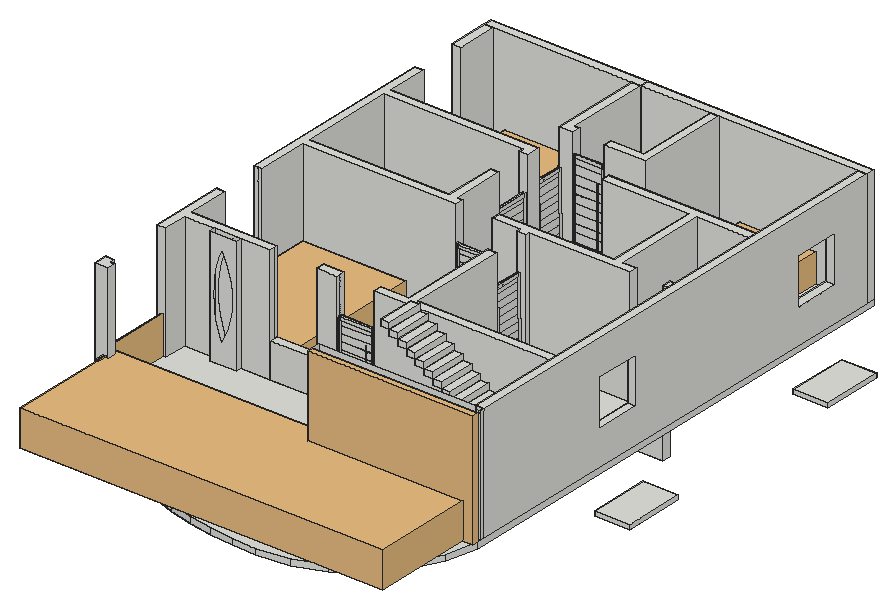
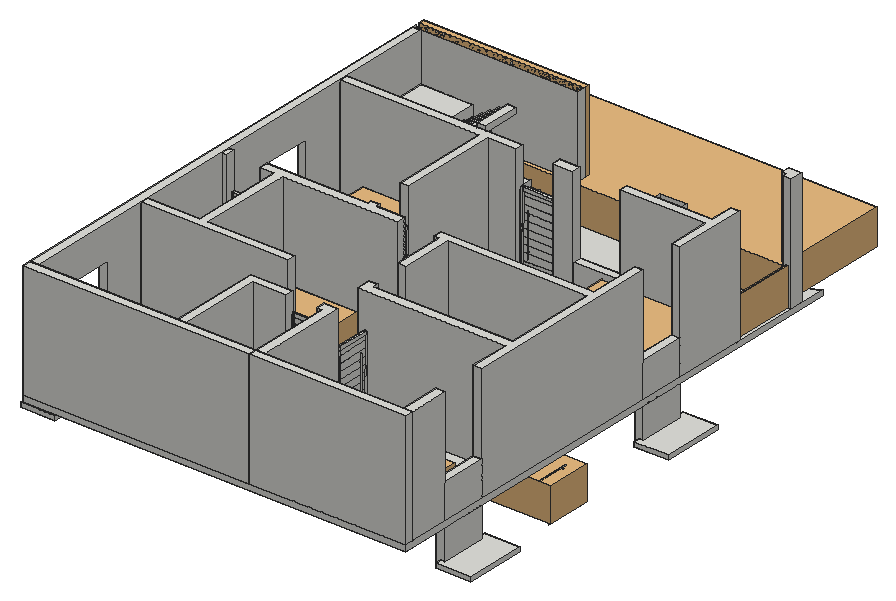
# SketchUp Ruby script. Lengths in inches.
U = 1.inch
M = Sketchup.active_model
def pt(a) = Geom::Point3d.new(a.map { |v| v * U })
def face(e, loops, mat)
  f = e.add_face(loops[0].map { |a| pt(a) })
  loops[1..].each { |l| e.add_face(l.map { |a| pt(a) }).erase! }
  f.material = f.back_material = mat if mat
  f
end
# faces: each face lists its corners as indices into pts; further lists are holes
def faces(e, pts, list, mat = nil) = list.each { |f| face(e, (f[0].is_a?(Array) ? f : [f]).map { |l| l.map { |i| pts[i] } }, mat) }
# xy, xz, yz: faces in a plane at the given z, y or x. An outline is a flat list of corners, or four numbers for a rectangle; further outlines are holes
def ring(l) = l.size == 4 ? [[l[0], l[1]], [l[2], l[1]], [l[2], l[3]], [l[0], l[3]]] : l.each_slice(2).to_a
def flat(e, list, mat, &to3) = list.each { |f| face(e, (f[0].is_a?(Array) ? f : [f]).map { |l| ring(l).map { |u, v| to3.(u, v) } }, mat) }
def xy(e, z, list, mat = nil) = flat(e, list, mat) { |x, y| [x, y, z] }
def xz(e, y, list, mat = nil) = flat(e, list, mat) { |x, z| [x, y, z] }
def yz(e, x, list, mat = nil) = flat(e, list, mat) { |y, z| [x, y, z] }
def lines(e, pts, list) = list.each { |a, b| e.add_line(pt(pts[a]), pt(pts[b])) }
# prism: a flat outline (further loops are holes) pulled along v
def prism(e, loops, v, mat = nil)
  f = face(e, loops, mat); d = Geom::Vector3d.new(v.map { |x| x * U })
  f.pushpull(f.normal.samedirection?(d) ? d.length : -d.length)
end
def box(e, o, s, mat = nil) = prism(e, [[o, [o[0] + s[0], o[1], o[2]], [o[0] + s[0], o[1] + s[1], o[2]], [o[0], o[1] + s[1], o[2]]]], [0, 0, s[2]], mat)
def at(x, y, z, deg = 0) = Geom::Transformation.translation(pt([x, y, z])) * Geom::Transformation.rotation(ORIGIN, Z_AXIS, deg.degrees)
def axes(o, x, y, z) = Geom::Transformation.new([*x, 0, *y, 0, *z, 0, *pt(o).to_a, 1])
def part(name) = M.definitions.add(name)
# library, detail: a bought-in or finely detailed component or shape, given as its bounding box
def library(name, o, s) = part(name).tap { |d| box(d.entities, o, s) }
def detail(e, o, s) = box(e.add_group.entities, o, s)
def put(e, d, t, mat = nil) = e.add_instance(d, t).tap { |i| i.material = mat if mat }
def group(e, t, mat = nil) = e.add_group.tap { |g| g.transformation = t; g.material = mat if mat }.entities
root = M.entities
c1 = part("Группа\#62")
xz(c1.entities,1.5625,[[-122.05,-1.18,-77.55,0]])
p = [[-122.05,0,0],[-122.05,1.5625,0]]
lines(c1.entities,p,[[0,1]])
c2 = part("Группа\#121")
xz(c2.entities,0,[[[0,0,3.9375,3.9375],[0.39,0.39,3.54,3.54]]])
p = [[0.39,0,0.39],[1.97,0.39,1.97],[3.54,0,0.39],[0.39,0,3.54],[3.54,0,3.54]]
faces(c2.entities,p,[[0,1,2],[0,3,1],[4,2,1],[4,1,3]])
c3 = part("Группа\#115")
xy(c3.entities,0,[[0,-1.97,3.9375,9.84]])
xy(c3.entities,7.875,[[0,-1.97,3.9375,13.78]])
xz(c3.entities,-1.97,[[0,0,3.9375,7.875]])
yz(c3.entities,0,[[-1.97,0,-1.97,7.875,13.78,7.875,13.78,3.9375,13.3,3.81,12.84,3.65,12.4,3.4375,11.98,3.18,11.58,2.89,11.22,2.56,10.89,2.19,10.6,1.8,10.34,1.38,10.13,0.9375,9.96,0.48,9.84,0]])
yz(c3.entities,3.9375,[[-1.97,0,9.84,0,9.96,0.48,10.13,0.9375,10.34,1.38,10.6,1.8,10.89,2.19,11.22,2.56,11.58,2.89,11.98,3.18,12.4,3.4375,12.84,3.65,13.3,3.81,13.78,3.9375,13.78,7.875,-1.97,7.875]])
p = [[0,9.84,0],[0,9.96,0.48],[3.9375,9.96,0.48],[3.9375,9.84,0],[0,10.13,0.9375],[3.9375,10.13,0.9375],
  [0,10.34,1.38],[3.9375,10.34,1.38],[0,10.6,1.8],[3.9375,10.6,1.8],[0,10.89,2.19],[3.9375,10.89,2.19],
  [0,11.22,2.56],[3.9375,11.22,2.56],[0,11.58,2.89],[3.9375,11.58,2.89],[0,11.98,3.18],[3.9375,11.98,3.18],
  [0,12.4,3.4375],[3.9375,12.4,3.4375],[0,12.84,3.65],[3.9375,12.84,3.65],[0,13.3,3.81],[3.9375,13.3,3.81],
  [0,13.78,3.9375],[3.9375,13.78,3.9375]]
faces(c3.entities,p,[[0,1,2,3],[1,4,5,2],[4,6,7,5],[6,8,9,7],[8,10,11,9],[10,12,13,11],[12,14,15,13],[14,16,17,15],
  [16,18,19,17],[18,20,21,19],[20,22,23,21],[22,24,25,23]])
put(c3.entities,c2,at(0,13.78,3.9375))
c4 = library("Группа\#83",[-9.65,-17.52,0],[19.3,35.04,0.98])
c5 = library("Группа\#64",[-11.61,-17.52,0],[23.22,35.04,0.98])
c6 = part("Группа\#82")
xy(c6.entities,0,[[[-5.71,-17.52,5.71,17.52],[-3.66,-15.47,3.66,15.47]]])
xy(c6.entities,0.49,[[-3.35,-15.16,3.35,15.16]])
xy(c6.entities,0.98,[[[-5.71,-17.52,5.71,17.52],[-3.66,-15.47,3.66,15.47]]])
xz(c6.entities,-17.52,[[-5.71,0,5.71,0.98]])
xz(c6.entities,-15.16,[[-3.35,0.31,3.35,0.49],[-3.35,0.49,3.35,0.67]])
xz(c6.entities,15.16,[[-3.35,0.31,3.35,0.49],[-3.35,0.49,3.35,0.67]])
xz(c6.entities,17.52,[[-5.71,0,5.71,0.98]])
yz(c6.entities,-5.71,[[-17.52,0,17.52,0.98]])
yz(c6.entities,-3.35,[[-15.16,0.31,15.16,0.49],[-15.16,0.49,15.16,0.67]])
yz(c6.entities,3.35,[[-15.16,0.31,15.16,0.49],[-15.16,0.49,15.16,0.67]])
yz(c6.entities,5.71,[[-17.52,0,17.52,0.98]])
p = [[-3.35,-15.16,0.31],[3.35,-15.16,0.31],[-3.66,-15.47,0],[-3.66,15.47,0],[3.66,-15.47,0],[3.35,15.16,0.31],
  [3.66,15.47,0],[-3.35,15.16,0.31],[-3.35,-15.16,0.67],[-3.35,15.16,0.67],[-3.66,-15.47,0.98],[3.66,-15.47,0.98],
  [-3.66,15.47,0.98],[3.35,-15.16,0.67],[3.35,15.16,0.67],[3.66,15.47,0.98]]
faces(c6.entities,p,[[0,1,2],[2,3,0],[2,1,4],[5,4,1],[6,4,5],[7,0,3],[3,6,7],[5,7,6],
  [8,9,10],[10,11,8],[10,9,12],[13,8,11],[14,13,11],[14,11,15],[15,12,9],[14,15,9]])
c7 = part("Группа\#67")
xy(c7.entities,0,[[[-5.51,-17.52,5.51,17.52],[-3.46,-15.47,3.46,15.47]]])
xy(c7.entities,0.49,[[-3.15,-15.16,3.15,15.16]])
xy(c7.entities,0.98,[[[-5.51,-17.52,5.51,17.52],[-3.46,-15.47,3.46,15.47]]])
xz(c7.entities,-17.52,[[-5.51,0,5.51,0.98]])
xz(c7.entities,-15.16,[[-3.15,0.31,3.15,0.49],[-3.15,0.49,3.15,0.67]])
xz(c7.entities,15.16,[[-3.15,0.31,3.15,0.49],[-3.15,0.49,3.15,0.67]])
xz(c7.entities,17.52,[[-5.51,0,5.51,0.98]])
yz(c7.entities,-5.51,[[-17.52,0,17.52,0.98]])
yz(c7.entities,-3.15,[[-15.16,0.31,15.16,0.49],[-15.16,0.49,15.16,0.67]])
yz(c7.entities,3.15,[[-15.16,0.31,15.16,0.49],[-15.16,0.49,15.16,0.67]])
yz(c7.entities,5.51,[[-17.52,0,17.52,0.98]])
p = [[-3.15,-15.16,0.31],[3.15,-15.16,0.31],[-3.46,-15.47,0],[-3.46,15.47,0],[3.46,-15.47,0],[3.15,15.16,0.31],
  [3.46,15.47,0],[-3.15,15.16,0.31],[-3.15,-15.16,0.67],[-3.15,15.16,0.67],[-3.46,-15.47,0.98],[3.46,-15.47,0.98],
  [-3.46,15.47,0.98],[3.15,-15.16,0.67],[3.15,15.16,0.67],[3.46,15.47,0.98]]
faces(c7.entities,p,[[0,1,2],[2,3,0],[2,1,4],[5,4,1],[6,4,5],[7,0,3],[3,6,7],[5,7,6],
  [8,9,10],[10,11,8],[10,9,12],[13,8,11],[14,13,11],[14,11,15],[15,12,9],[14,15,9]])
c8 = part("Группа\#71")
xy(c8.entities,0,[[-3.05,-15.16,3.05,15.16]])
c9 = part("Group\#141")
box(c9.entities,[0,0,0],[37.68,9,36.625])
c10 = part("Group\#14")
xy(c10.entities,36,[[0,0,9,48]])
yz(c10.entities,0,[[0,0,48,36]])
yz(c10.entities,9,[[0,0,48,36]])
c11 = part("Group\#15")
xy(c11.entities,0,[[0,0,9,48]])
xz(c11.entities,0,[[0,0,9,36]])
xz(c11.entities,48,[[0,0,9,36]])
put(c11.entities,c10,at(0,0,0))
c12 = part("Group\#17")
box(c12.entities,[0,0,0],[36,62.875,4.625])
c13 = library("Group\#5",[0,0,0],[3.15,94.04,36])
c14 = part("Agrupar\#4")
xy(c14.entities,0,[[0,0,60.82,4.875]])
c15 = part("Agrupar\#7")
box(c15.entities,[0,0,0.25],[0.65,5.875,0.35])
c16 = part("Agrupar\#15")
prism(c16.entities,[[[0,0.625,0],[0.65,0.625,0],[0.65,0,0],[0,0,0]]],[0,0.02,45.16])
c17 = part("Agrupar\#14")
put(c17.entities,c15,at(0,0.65,6.88))
put(c17.entities,c16,at(0,0,0))
put(c17.entities,c15,at(0,0.65,40.25))
c18 = part("Agrupar\#6")
prism(c18.entities,[[[-0.5,0.62,-4.9375],[0.77,0.62,-4.9375],[0.77,-0.19,-4.9375],[-0.5,-0.19,-4.9375]]],[0,0.03,52.91])
c19 = part("Agrupar\#8")
put(c19.entities,c15,at(0,0.65,6.88))
put(c19.entities,c18,at(0,0,0))
put(c19.entities,c15,at(0,0.65,40.25))
c20 = part("Agrupar\#2")
prism(c20.entities,[[[0,2.67,0.04],[55.46,2.67,0.04],[55.46,0.04,0],[0,0.04,0]]],[0,-0.04,3.23])
c21 = part("Agrupar\#10")
prism(c21.entities,[[[0,3.76,0.04],[4.23,3.76,0.04],[4.23,1.14,0],[0,1.14,0]]],[0,-1.14,83.14])
c22 = part("Agrupar\#1")
prism(c22.entities,[[[0,3.76,0.04],[4.23,3.76,0.04],[4.23,1.14,0],[0,1.14,0]]],[0,-1.14,83.14])
c23 = part("Agrupar\#3")
put(c23.entities,c20,at(4.23,0,79.91))
put(c23.entities,c21,at(59.6875,0,0))
put(c23.entities,c22,at(0,0,0))
c24 = part("Agrupar\#5")
put(c24.entities,c23,axes([0,-1.34,0.11],[1,0,0],[0,3.10443,-0.05961],[0,0.0192,0.99982]))
c25 = part("Agrupar\#9")
put(c25.entities,c17,axes([49.36,10.72,17.77],[1,0,0],[0,-1,0],[0,0,1]))
put(c25.entities,c19,at(49.36,0,17.76))
put(c25.entities,c24,at(0,0.21,0.01))
c26 = part("Agrupar\#11")
box(c26.entities,[0,0,0],[60.82,4.875,7.44])
c27 = part("Agrupar\#12")
put(c27.entities,c26,at(0,0,67.34))
put(c27.entities,c26,at(0,0,44.83))
put(c27.entities,c26,at(0,0,59.9))
put(c27.entities,c26,at(0,0,74.78))
put(c27.entities,c26,at(0,0,52.37))
put(c27.entities,c26,at(0,0,7.53))
put(c27.entities,c26,at(0,0,0))
put(c27.entities,c26,at(0,0,29.95))
put(c27.entities,c26,at(0,0,15.07))
put(c27.entities,c26,at(0,0,22.51))
put(c27.entities,c26,at(0,0,37.39))
c28 = part("Agrupar\#13")
put(c28.entities,c25,at(0,0,0.0625))
put(c28.entities,c27,axes([2.375,5.17,0.15],[1,0,0],[0,0.48232,0.01095],[0,-0.02269,0.99974]))
c29 = part("PORTA PIVOTANDE ENVERNIZADA LUXURY")
p = [[59.6875,-1.28,79.91],[59.6875,-3.1,79.89],[4.23,-1.28,79.91],[4.23,-3.1,79.89]]
lines(c29.entities,p,[[0,1],[2,3]])
put(c29.entities,c14,at(0.13,-2.89,82.23))
put(c29.entities,c28,at(0,-6.8,-0.11))
c30 = library("bed",[0,0,0],[81.24,78.82,29.53])
c31 = library("Group\#4",[0,0,0],[375.02,122.21,36.98])
c32 = library("Group\#236",[0,0,0],[3.15,9.6875,36.98])
c33 = library("Group\#213",[0,0,1.6875],[171,5.375,120])
c34 = library("SOFAS",[-9.33,-51.94,0],[132.18,168.58,37.5625])
c35 = library("Group\#169",[0,0,0],[83.17,58.86,38.65])
c36 = part("Group\#19")
box(c36.entities,[0,0,0],[9,39,6])
c37 = part("Group\#20")
box(c37.entities,[0,0,0],[54,96,10])
c38 = part("Группа\#53")
xy(c38.entities,0,[[[-6.3,-13.1875,6.3,13.1875],[-4.25,-11.14,4.25,11.14]]])
xy(c38.entities,0.49,[[-3.9375,-10.83,3.9375,10.83]])
xy(c38.entities,0.98,[[[-6.3,-13.1875,6.3,13.1875],[-4.25,-11.14,4.25,11.14]]])
xz(c38.entities,-13.1875,[[-6.3,0,6.3,0.98]])
xz(c38.entities,-10.83,[[-3.9375,0.31,3.9375,0.49],[-3.9375,0.49,3.9375,0.67]])
xz(c38.entities,10.83,[[-3.9375,0.31,3.9375,0.49],[-3.9375,0.49,3.9375,0.67]])
xz(c38.entities,13.1875,[[-6.3,0,6.3,0.98]])
yz(c38.entities,-6.3,[[-13.1875,0,13.1875,0.98]])
yz(c38.entities,-3.9375,[[-10.83,0.31,10.83,0.49],[-10.83,0.49,10.83,0.67]])
yz(c38.entities,3.9375,[[-10.83,0.31,10.83,0.49],[-10.83,0.49,10.83,0.67]])
yz(c38.entities,6.3,[[-13.1875,0,13.1875,0.98]])
p = [[-3.9375,-10.83,0.31],[3.9375,-10.83,0.31],[-4.25,-11.14,0],[-4.25,11.14,0],[4.25,-11.14,0],[4.25,11.14,0],
  [-3.9375,10.83,0.31],[3.9375,10.83,0.31],[-3.9375,-10.83,0.67],[-3.9375,10.83,0.67],[-4.25,-11.14,0.98],[4.25,-11.14,0.98],
  [-4.25,11.14,0.98],[3.9375,-10.83,0.67],[3.9375,10.83,0.67],[4.25,11.14,0.98]]
faces(c38.entities,p,[[0,1,2],[2,3,0],[2,1,4],[5,4,1],[6,0,3],[7,5,1],[3,5,6],[7,6,5],
  [8,9,10],[10,11,8],[10,9,12],[13,8,11],[14,13,11],[14,11,15],[15,12,9],[14,15,9]])
c39 = part("Группа\#13")
xy(c39.entities,0,[[0,0,21.73,35.43]])
xy(c39.entities,29.92,[[0,0,21.73,35.43]])
xz(c39.entities,0,[[0,0,21.73,29.92]])
xz(c39.entities,35.43,[[0,0,21.73,29.92]])
yz(c39.entities,0,[[0,0,35.43,29.92]])
yz(c39.entities,21.73,[[0,0,22.44,29.92],[22.44,0,35.43,3.15],[[22.44,3.15,35.43,29.92],[22.64,3.35,35.24,29.72]]])
put(c39.entities,c38,axes([21.46,28.9375,16.54],[0,1,0],[0,0,1],[1,0,0]))
c40 = library("LIXEIRA INOX DE BANHEIRO",[-4.13,-4.13,0],[8.25,8.24,13.39])
c41 = part("Группа\#59")
xy(c41.entities,0,[[-13.1875,-4.13,13.1875,4.13]])
c42 = part("Panelled cabinet front \#2")
xy(c42.entities,0,[[[-15.55,-6.5,15.55,6.5],[-13.5,-4.45,13.5,4.45]]])
xy(c42.entities,0.98,[[[-15.55,-6.5,15.55,6.5],[-13.5,-4.45,13.5,4.45]]])
xz(c42.entities,-6.5,[[-15.55,0,15.55,0.98]])
xz(c42.entities,-4.13,[[-13.1875,0.31,13.1875,0.67]])
xz(c42.entities,4.13,[[-13.1875,0.31,13.1875,0.67]])
xz(c42.entities,6.5,[[-15.55,0,15.55,0.98]])
yz(c42.entities,-15.55,[[-6.5,0,6.5,0.98]])
yz(c42.entities,-13.1875,[[-4.13,0.31,4.13,0.67]])
yz(c42.entities,13.1875,[[-4.13,0.31,4.13,0.67]])
yz(c42.entities,15.55,[[-6.5,0,6.5,0.98]])
p = [[13.5,-4.45,0],[-13.5,-4.45,0],[13.1875,-4.13,0.31],[-13.1875,-4.13,0.31],[-13.1875,4.13,0.31],[-13.5,4.45,0],
  [13.1875,4.13,0.31],[13.5,4.45,0],[-13.5,4.45,0.98],[-13.5,-4.45,0.98],[-13.1875,-4.13,0.67],[13.5,-4.45,0.98],
  [13.1875,-4.13,0.67],[13.5,4.45,0.98],[-13.1875,4.13,0.67],[13.1875,4.13,0.67]]
faces(c42.entities,p,[[0,1,2],[3,2,1],[4,3,1],[1,5,4],[2,6,0],[0,6,7],[7,4,5],[6,4,7],
  [8,9,10],[11,10,9],[12,10,11],[11,13,12],[10,14,8],[15,12,13],[14,13,8],[14,15,13]])
put(c42.entities,c41,at(0,0,0.49))
c43 = part("Группа\#3")
xy(c43.entities,0,[[[-7.68,-13.1875,7.68,13.1875],[-5.63,-11.14,5.63,11.14]]])
xy(c43.entities,0.49,[[-5.31,-10.83,5.31,10.83]])
xy(c43.entities,0.98,[[[-7.68,-13.1875,7.68,13.1875],[-5.63,-11.14,5.63,11.14]]])
xz(c43.entities,-13.1875,[[-7.68,0,7.68,0.98]])
xz(c43.entities,-10.83,[[-5.31,0.31,5.31,0.49],[-5.31,0.49,5.31,0.67]])
xz(c43.entities,10.83,[[-5.31,0.31,5.31,0.49],[-5.31,0.49,5.31,0.67]])
xz(c43.entities,13.1875,[[-7.68,0,7.68,0.98]])
yz(c43.entities,-7.68,[[-13.1875,0,13.1875,0.98]])
yz(c43.entities,-5.31,[[-10.83,0.31,10.83,0.49],[-10.83,0.49,10.83,0.67]])
yz(c43.entities,5.31,[[-10.83,0.31,10.83,0.49],[-10.83,0.49,10.83,0.67]])
yz(c43.entities,7.68,[[-13.1875,0,13.1875,0.98]])
p = [[-5.31,-10.83,0.31],[5.31,-10.83,0.31],[-5.63,-11.14,0],[-5.63,11.14,0],[5.63,-11.14,0],[5.63,11.14,0],
  [-5.31,10.83,0.31],[5.31,10.83,0.31],[-5.31,-10.83,0.67],[-5.31,10.83,0.67],[-5.63,-11.14,0.98],[5.63,-11.14,0.98],
  [-5.63,11.14,0.98],[5.31,-10.83,0.67],[5.31,10.83,0.67],[5.63,11.14,0.98]]
faces(c43.entities,p,[[0,1,2],[2,3,0],[2,1,4],[5,4,1],[6,0,3],[7,5,1],[3,5,6],[7,6,5],
  [8,9,10],[10,11,8],[10,9,12],[13,8,11],[14,13,11],[14,11,15],[15,12,9],[14,15,9]])
c44 = part("Panelled cabinet front \#1")
xy(c44.entities,0,[[[-7.68,-13.1875,7.68,13.1875],[-5.63,-11.14,5.63,11.14]]])
xy(c44.entities,0.49,[[-5.31,-10.83,5.31,10.83]])
xy(c44.entities,0.98,[[[-7.68,-13.1875,7.68,13.1875],[-5.63,-11.14,5.63,11.14]]])
xz(c44.entities,-13.1875,[[-7.68,0,7.68,0.98]])
xz(c44.entities,-10.83,[[-5.31,0.31,5.31,0.49],[-5.31,0.49,5.31,0.67]])
xz(c44.entities,10.83,[[-5.31,0.31,5.31,0.49],[-5.31,0.49,5.31,0.67]])
xz(c44.entities,13.1875,[[-7.68,0,7.68,0.98]])
yz(c44.entities,-7.68,[[-13.1875,0,13.1875,0.98]])
yz(c44.entities,-5.31,[[-10.83,0.31,10.83,0.49],[-10.83,0.49,10.83,0.67]])
yz(c44.entities,5.31,[[-10.83,0.31,10.83,0.49],[-10.83,0.49,10.83,0.67]])
yz(c44.entities,7.68,[[-13.1875,0,13.1875,0.98]])
p = [[-5.31,-10.83,0.31],[5.31,-10.83,0.31],[-5.63,-11.14,0],[-5.63,11.14,0],[5.63,-11.14,0],[5.63,11.14,0],
  [-5.31,10.83,0.31],[5.31,10.83,0.31],[-5.63,-11.14,0.98],[5.63,-11.14,0.98],[-5.31,-10.83,0.67],[-5.31,10.83,0.67],
  [-5.63,11.14,0.98],[5.31,-10.83,0.67],[5.31,10.83,0.67],[5.63,11.14,0.98]]
faces(c44.entities,p,[[0,1,2],[2,3,0],[2,1,4],[5,4,1],[6,0,3],[7,5,1],[3,5,6],[7,6,5],
  [8,9,10],[10,11,8],[8,11,12],[13,10,9],[14,13,9],[14,9,15],[15,12,11],[14,15,11]])
c45 = part("Группа\#8")
xy(c45.entities,0,[[[-5.71,-13.1875,5.71,13.1875],[-3.66,-11.14,3.66,11.14]]])
xy(c45.entities,0.49,[[-3.35,-10.83,3.35,10.83]])
xy(c45.entities,0.98,[[[-5.71,-13.1875,5.71,13.1875],[-3.66,-11.14,3.66,11.14]]])
xz(c45.entities,-13.1875,[[-5.71,0,5.71,0.98]])
xz(c45.entities,-10.83,[[-3.35,0.31,3.35,0.49],[-3.35,0.49,3.35,0.67]])
xz(c45.entities,10.83,[[-3.35,0.31,3.35,0.49],[-3.35,0.49,3.35,0.67]])
xz(c45.entities,13.1875,[[-5.71,0,5.71,0.98]])
yz(c45.entities,-5.71,[[-13.1875,0,13.1875,0.98]])
yz(c45.entities,-3.35,[[-10.83,0.31,10.83,0.49],[-10.83,0.49,10.83,0.67]])
yz(c45.entities,3.35,[[-10.83,0.31,10.83,0.49],[-10.83,0.49,10.83,0.67]])
yz(c45.entities,5.71,[[-13.1875,0,13.1875,0.98]])
p = [[3.66,-11.14,0],[-3.66,-11.14,0],[-3.35,-10.83,0.31],[-3.66,11.14,0],[3.35,-10.83,0.31],[3.66,11.14,0],
  [-3.35,10.83,0.31],[3.35,10.83,0.31],[-3.66,11.14,0.98],[-3.66,-11.14,0.98],[-3.35,10.83,0.67],[-3.35,-10.83,0.67],
  [3.35,-10.83,0.67],[3.66,-11.14,0.98],[3.35,10.83,0.67],[3.66,11.14,0.98]]
faces(c45.entities,p,[[0,1,2],[3,2,1],[4,0,2],[5,0,4],[6,2,3],[7,5,4],[3,5,6],[7,6,5],
  [8,9,10],[11,10,9],[12,11,9],[12,9,13],[14,12,13],[13,15,14],[10,14,8],[8,14,15]])
c46 = part("Группа\#15")
xy(c46.entities,0,[[[-6.4,-13.1875,6.4,13.1875],[-4.35,-11.14,4.35,11.14]]])
xy(c46.entities,0.49,[[-4.04,-10.83,4.04,10.83]])
xy(c46.entities,0.98,[[[-6.4,-13.1875,6.4,13.1875],[-4.35,-11.14,4.35,11.14]]])
xz(c46.entities,-13.1875,[[-6.4,0,6.4,0.98]])
xz(c46.entities,-10.83,[[-4.04,0.31,4.04,0.49],[-4.04,0.49,4.04,0.67]])
xz(c46.entities,10.83,[[-4.04,0.31,4.04,0.49],[-4.04,0.49,4.04,0.67]])
xz(c46.entities,13.1875,[[-6.4,0,6.4,0.98]])
yz(c46.entities,-6.4,[[-13.1875,0,13.1875,0.98]])
yz(c46.entities,-4.04,[[-10.83,0.31,10.83,0.49],[-10.83,0.49,10.83,0.67]])
yz(c46.entities,4.04,[[-10.83,0.31,10.83,0.49],[-10.83,0.49,10.83,0.67]])
yz(c46.entities,6.4,[[-13.1875,0,13.1875,0.98]])
p = [[4.35,-11.14,0],[-4.35,-11.14,0],[-4.04,-10.83,0.31],[-4.04,10.83,0.31],[-4.35,11.14,0],[4.04,-10.83,0.31],
  [4.35,11.14,0],[4.04,10.83,0.31],[-4.35,11.14,0.98],[-4.35,-11.14,0.98],[-4.04,-10.83,0.67],[4.35,-11.14,0.98],
  [4.04,-10.83,0.67],[4.35,11.14,0.98],[-4.04,10.83,0.67],[4.04,10.83,0.67]]
faces(c46.entities,p,[[0,1,2],[3,2,1],[1,4,3],[5,0,2],[6,0,7],[5,7,0],[6,3,4],[7,3,6],
  [8,9,10],[11,10,9],[12,10,11],[13,12,11],[10,14,8],[15,12,13],[13,8,15],[14,15,8]])
c47 = part("Группа\#5")
xy(c47.entities,0,[[-13.1875,-4.13,13.1875,4.13]])
c48 = library("Inodoro ROCA Meridian-N compact",[-14.68,0,0],[14.68,23.62,31.16])
c49 = library("Grupo\#9",[0.45,21.05,9.1],[4.32,4.21,6.93])
box(root,[428.25,528.25,84],[36,62.875,4.625])
box(root,[428.25,271.75,84],[36,62.875,4.625])
xy(root,126,[[257.25,124.9375,428.25,129],[72.5,219,99.9375,225]])
xz(root,120,[[257.25,126,275.57,127.6,293.66,130.93,311.34,135.98,328.47,142.6875,344.87,151,360.41,160.83,374.95,172.1,388.34,184.7,400.47,198.53,411.23,213.44,420.52,229.3125,428.25,246,257.25,246]])
xz(root,124.9375,[[257.25,126,428.25,126,428.25,246,420.52,229.3125,411.23,213.44,400.47,198.53,388.34,184.7,374.95,172.1,360.41,160.83,344.87,151,328.47,142.6875,311.34,135.98,293.66,130.93,275.57,127.6]])
xz(root,129,[[257.25,126,428.25,246]])
xz(root,141.125,[[275.25,120,419.25,126]])
xz(root,219,[[[72.5,126,99.9375,246],[84.13,145.18,81.6,152.25,79.51,159.47,77.87,166.8,76.7,174.22,75.99,181.7,75.76,189.21,75.99,196.72,76.7,204.2,77.87,211.625,79.51,218.96,81.6,226.17,84.13,233.24,87.67,226.43,90.6,219.33,92.9,212,94.55,204.5,95.55,196.89,95.88,189.21,95.55,181.54,94.55,173.93,92.9,166.43,90.6,159.1,87.67,152]]])
xz(root,225,[[275.25,120,419.25,126],[[72.5,126,99.9375,246],[84.13,145.18,87.67,152,90.6,159.1,92.9,166.43,94.55,173.93,95.55,181.54,95.88,189.21,95.55,196.89,94.55,204.5,92.9,212,90.6,219.33,87.67,226.43,84.13,233.24,81.6,226.17,79.51,218.96,77.87,211.625,76.7,204.2,75.99,196.72,75.76,189.21,75.99,181.7,76.7,174.22,77.87,166.8,79.51,159.47,81.6,152.25]]])
xz(root,422.43,[[41.25,126,62.98,129.15],[41.25,129.15,62.98,155.92]])
xz(root,534,[[32.25,126,41.25,162]])
xz(root,582,[[32.25,126,41.25,162]])
yz(root,62.98,[[[422.43,129.15,434.24,155.92],[422.63,129.35,434.05,155.72]]])
yz(root,72.5,[[219,126,225,246]])
yz(root,99.9375,[[219,126,225,246]])
yz(root,257.25,[[120,126,129,246]])
yz(root,275.25,[[141.125,120,225,126]])
yz(root,419.25,[[141.125,120,225,126]])
yz(root,428.25,[[124.9375,126,129,246]])
p = [[275.57,120,127.6],[257.25,120,126],[257.25,124.9375,126],[275.57,124.9375,127.6],[293.66,120,130.93],[293.66,124.9375,130.93],
  [311.34,120,135.98],[311.34,124.9375,135.98],[328.47,120,142.6875],[328.47,124.9375,142.6875],[41.25,624,126],[41.25,624,246],
  [32.25,624,126],[32.25,624,246],[199.25,225,120],[199.25,225,83.375],[236.93,225,83.375],[236.93,225,120],
  [41.25,624,120],[32.25,624,120],[53.0625,410.82,90.35],[53.0625,410.82,55.31],[53.0625,434.05,90.35],[53.0625,434.05,55.31],
  [163.51,398.8125,90.55],[163.44,399.06,90.55]]
faces(root,p,[[0,1,2,3],[4,0,3,5],[6,4,5,7],[8,6,7,9]])
lines(root,p,[[10,11],[12,13],[14,15],[16,17],[15,16],[18,19],[20,21],[22,20],[23,22],[21,23],[24,25]])
detail(root,[41.25,387,55.12],[122.55,47.24,35.43])
detail(root,[96.99,399.52,55.78],[1.27,1.56,1.27])
detail(root,[94.48,399.52,55.78],[1.27,1.56,1.27])
detail(root,[74.68,399.52,55.91],[1.27,1.56,1.27])
detail(root,[53.77,411.36,55.95],[1.56,1.28,1.28])
detail(root,[62.98,387,126],[123.94,23.56,29.92])
put(root,c1,at(40.71,312.33,55.12,-90))
put(root,c3,at(158.18,387.79,55.12))
put(root,c3,at(117.23,387.79,55.12))
put(root,c4,axes([106.21,398.54,72.83],[1,0,0],[0,0,1],[0,1,0]))
put(root,c4,axes([86.53,398.54,72.83],[-1,0,0],[0,0,1],[0,1,0]))
put(root,c5,axes([52.79,422.43,72.83],[0,1,0],[0,0,1],[1,0,0]))
put(root,c6,axes([70.78,398.54,72.83],[-1,0,0],[0,0,1],[0,1,0]))
put(root,c7,axes([52.79,405.13,72.83],[0,0.96,0],[0,0,1],[1,0,0]))
put(root,c8,axes([59.26,399.03,72.83],[-1,0,0],[0,0,1],[0,1,0]))
g1 = group(root,at(414.25,387,83.375))
box(g1,[-34.5,-9,0],[34.5,9,36.625])
put(root,c9,axes([185.25,529.3125,83.375],[0,-0.99033,0],[1,0,0],[0,0,1]))
put(root,c9,axes([185.25,478,83.375],[0,-0.99033,0],[1,0,0],[0,0,1]))
put(root,c9,at(266.25,373.5,83.375,-90))
put(root,c9,at(199.25,225,83.375))
put(root,c9,at(199.58,378,83.375))
put(root,c11,at(177.75,225,84,90))
put(root,c11,at(32.25,277.5,84))
put(root,c11,at(32.25,534,84))
put(root,c12,at(0,525.84,84.03))
put(root,c12,at(0,269.34,84.03))
g2 = group(root,at(32.25,0,120))
xy(g2,0,[[[262.875,0,295.28,3.98,325.75,15.69,352.49,34.43,373.89,59.08,388.6875,88.18,396,120,396,633,0,633,0,93.38,1.84,94.89,3.86,96.16,6.02,97.17,8.29,97.9,10.63,98.34,13.01,98.49,15.38,98.34,17.73,97.9,19.99,97.17,22.15,96.16,24.17,94.89,26.01,93.38,35.1,84.92,54.44,69.35,74.83,55.19,96.1875,42.53,118.39,31.42,141.33,21.92,164.89,14.08,188.94,7.95,213.38,3.54,238.0625,0.89],[243,141.125,387,225]]])
xy(g2,6,[[[262.875,0,295.28,3.98,325.75,15.69,352.49,34.43,373.89,59.08,388.6875,88.18,396,120,396,633,0,633,0,93.38,1.84,94.89,3.86,96.16,6.02,97.17,8.29,97.9,10.63,98.34,13.01,98.49,15.38,98.34,17.73,97.9,19.99,97.17,22.15,96.16,24.17,94.89,26.01,93.38,35.1,84.92,54.44,69.35,74.83,55.19,96.1875,42.53,118.39,31.42,141.33,21.92,164.89,14.08,188.94,7.95,213.38,3.54,238.0625,0.89],[243,141.125,387,225]]])
xz(g2,633,[[0,0,396,6]])
yz(g2,0,[[93.38,0,633,6]])
yz(g2,396,[[120,0,633,6]])
p = [[262.875,0,6],[238.0625,0.89,6],[238.0625,0.89,0],[262.875,0,0],[295.28,3.98,6],[295.28,3.98,0],
  [213.38,3.54,6],[213.38,3.54,0],[188.94,7.95,6],[188.94,7.95,0],[325.75,15.69,6],[325.75,15.69,0],
  [164.89,14.08,6],[164.89,14.08,0],[141.33,21.92,6],[141.33,21.92,0],[352.49,34.43,6],[352.49,34.43,0],
  [118.39,31.42,6],[118.39,31.42,0],[96.1875,42.53,6],[96.1875,42.53,0],[373.89,59.08,6],[373.89,59.08,0],
  [74.83,55.19,6],[74.83,55.19,0],[54.44,69.35,6],[54.44,69.35,0],[388.6875,88.18,6],[388.6875,88.18,0],
  [35.1,84.92,6],[35.1,84.92,0],[26.01,93.38,6],[26.01,93.38,0],[396,120,6],[396,120,0],
  [1.84,94.89,6],[0,93.38,6],[0,93.38,0],[1.84,94.89,0],[24.17,94.89,6],[24.17,94.89,0],
  [3.86,96.16,6],[3.86,96.16,0],[22.15,96.16,6],[22.15,96.16,0],[6.02,97.17,6],[6.02,97.17,0],
  [19.99,97.17,6],[19.99,97.17,0],[8.29,97.9,6],[8.29,97.9,0],[17.73,97.9,6],[17.73,97.9,0],
  [10.63,98.34,6],[10.63,98.34,0],[15.38,98.34,6],[15.38,98.34,0],[13.01,98.49,6],[13.01,98.49,0]]
faces(g2,p,[[0,1,2,3],[4,0,3,5],[1,6,7,2],[6,8,9,7],[10,4,5,11],[8,12,13,9],[12,14,15,13],[16,10,11,17],
  [14,18,19,15],[18,20,21,19],[22,16,17,23],[20,24,25,21],[24,26,27,25],[28,22,23,29],[26,30,31,27],[30,32,33,31],
  [34,28,29,35],[36,37,38,39],[32,40,41,33],[42,36,39,43],[40,44,45,41],[46,42,43,47],[44,48,49,45],[50,46,47,51],
  [48,52,53,49],[54,50,51,55],[52,56,57,53],[58,54,55,59],[56,58,59,57]])
put(root,c13,axes([35.45,134.16,125.79],[0.728,0,0],[0,0.728,0],[0,0,1.08472]))
put(root,c29,axes([186.83,529.3125,126.11],[0,-0.5895,0],[0.36,0,0],[0,0,1]))
put(root,c30,at(395.25,234,126,90))
g3 = group(root,at(32.25,120,126))
prism(g3,[[[14,0,0],[0,0,0],[0,14,0],[9,14,0],[9,9,0],[14,9,0]]],[0,0,120])
g4 = group(root,at(185.25,529.3125,126))
xy(g4,0,[[0,0,0,94.6875,9,94.6875,9,9,14,9,14,0],[46.9375,0,46.9375,8.8125,81,8.8125,81,94.6875,90,94.6875,90,0]])
xy(g4,120,[[0,0,14,0,14,9,9,9,9,94.6875,0,94.6875],[46.9375,0,90,0,90,94.6875,81,94.6875,81,8.8125,46.9375,8.8125]])
xz(g4,0,[[0,0,14,120],[46.9375,0,90,120]])
xz(g4,8.8125,[[46.9375,0,81,120]])
xz(g4,9,[[9,0,14,120]])
xz(g4,94.6875,[[0,0,9,120],[81,0,90,120]])
yz(g4,0,[[0,0,94.6875,120]])
yz(g4,9,[[9,0,94.6875,120]])
yz(g4,14,[[0,0,9,120]])
yz(g4,46.9375,[[0,0,8.8125,120]])
yz(g4,81,[[8.8125,0,94.6875,120]])
yz(g4,90,[[0,0,94.6875,120]])
put(root,c31,at(42.47,11.02,126))
put(root,c32,at(40.1875,110.8125,126))
put(root,c29,axes([199.25,530.13,126.18],[0.51535,0,0],[0,0.10352,0],[0,0,1.21]))
put(root,c33,at(257.25,114.625,124.3125))
put(root,c30,at(53.35,624,126,-90))
put(root,c30,at(296.25,624,126,-90))
put(root,c29,axes([273.28,529.68,126.15],[0,-0.5895,0],[0.36,0,0],[0,0,1]))
put(root,c29,axes([199.25,227.85,126.15],[0.5895,0,0],[0,0.36,0],[0,0,1]))
put(root,c29,axes([269.1,373.5,126.15],[0,-0.5895,0],[0.36,0,0],[0,0,1]))
put(root,c29,axes([379.75,380.94,126.15],[0.5398,0,0],[0,0.37131,0],[0,0,1]))
put(root,c34,axes([140.76,333.63,126],[-0.81,0,0],[0,-0.85419,0],[0,0,0.81]))
put(root,c29,axes([199.25,380.28,126.15],[0.5895,0,0],[0,0.36,0],[0,0,1]))
put(root,c29,axes([190.88,478.36,126.15],[0,-0.5895,0],[0.36,0,0],[0,0,1]))
g5 = group(root,at(236.93,225,126))
xy(g5,0,[[0,0,0,9,29.32,9,29.32,110.82,38.32,110.82,38.32,9,182.32,9,182.32,0]])
xy(g5,120,[[0,0,182.32,0,182.32,9,38.32,9,38.32,110.82,29.32,110.82,29.32,9,0,9]])
xz(g5,0,[[0,0,182.32,120]])
xz(g5,9,[[0,0,29.32,120],[38.32,0,182.32,120]])
xz(g5,110.82,[[29.32,0,38.32,120]])
yz(g5,0,[[0,0,9,120]])
yz(g5,29.32,[[9,0,110.82,120]])
yz(g5,38.32,[[9,0,110.82,120]])
yz(g5,182.32,[[0,0,9,120]])
put(root,c35,at(260,410.61,126))
g6 = group(root,at(32.25,201,126))
prism(g6,[[[9,76.5,0],[9,33,0],[97.5,33,0],[97.5,28.5,0],[97.5,24,0],[9,24,0],[9,0,0],[0,0,0],[0,76.5,0]]],[0,0,120])
g7 = group(root,at(275.25,129,126))
put(g7,c36,at(0,57,118))
put(g7,c36,at(63,57,76))
put(g7,c36,at(81,57,64))
put(g7,c36,at(0,0,0))
put(g7,c36,at(18,0,12))
put(g7,c36,at(9,0,6))
put(g7,c36,at(36,0,24))
put(g7,c36,at(27,0,18))
put(g7,c36,at(81,0,54))
put(g7,c36,at(72,57,70))
put(g7,c36,at(45,57,88))
put(g7,c36,at(72,0,48))
put(g7,c36,at(54,0,36))
put(g7,c36,at(27,57,100))
put(g7,c36,at(18,57,106))
put(g7,c36,at(9,57,112))
put(g7,c36,at(63,0,42))
put(g7,c37,at(90,0,60))
put(g7,c36,at(45,0,30))
put(g7,c36,at(54,57,82))
put(g7,c36,at(36,57,94))
g8 = group(root,at(177.75,225,126))
prism(g8,[[[21.5,0,0],[0,0,0],[0,9,0],[21.5,9,0],[21.5,2.72,0]]],[0,0,120])
put(root,c39,at(41.25,387,126))
g9 = group(root,at(177.75,225,126,90))
xy(g9,0,[[0,0,9,48]])
xz(g9,0,[[0,0,9,36]])
xz(g9,48,[[0,0,9,36]])
put(g9,c10,at(0,0,0))
g10 = group(root,at(32.25,534,126))
xy(g10,0,[[0,0,9,48]])
xz(g10,0,[[0,0,9,36]])
xz(g10,48,[[0,0,9,36]])
put(g10,c10,at(0,0,0))
g11 = group(root,at(419.25,129,126))
prism(g11,[[[0,495,0],[0,0,0],[0,0,120],[0,495,120]],[[0,405,84],[0,405,36],[0,453,36],[0,453,84]],[[0,196.5,36],[0,196.5,84],[0,148.5,84],[0,148.5,36]]],[9,0,0])
g12 = group(root,at(32.25,277.5,126))
xy(g12,0,[[0,0,9,48]])
xz(g12,0,[[0,0,9,36]])
xz(g12,48,[[0,0,9,36]])
put(g12,c10,at(0,0,0))
g13 = group(root,at(32.25,582,126))
box(g13,[0,0,0],[9,42,120])
g14 = group(root,at(266.25,624,126))
box(g14,[-72,0,0],[234,9,120])
g15 = group(root,at(32.25,325.5,126))
xy(g15,0,[[0,0,9,208.5],[9,52.5,9,61.5,153,61.5,153,115.1875,162,115.1875,162,61.5,167,61.5,167,52.5],[153,152.5,153,157.5,9,157.5,9,166.5,162,166.5,162,152.5]])
xy(g15,120,[[0,0,9,0,9,52.5,167,52.5,167,61.5,162,61.5,162,115.1875,153,115.1875,153,61.5,9,61.5,9,157.5,153,157.5,153,152.5,162,152.5,162,166.5,9,166.5,9,208.5,0,208.5]])
xz(g15,0,[[0,0,4.5,120],[4.5,0,9,120]])
xz(g15,52.5,[[9,0,167,120]])
xz(g15,61.5,[[9,0,153,120],[162,0,167,120]])
xz(g15,115.1875,[[153,0,162,120]])
xz(g15,152.5,[[153,0,162,120]])
xz(g15,157.5,[[9,0,153,120]])
xz(g15,166.5,[[9,0,162,120]])
xz(g15,208.5,[[0,0,9,120]])
yz(g15,0,[[0,0,208.5,120]])
yz(g15,9,[[0,0,52.5,120],[61.5,0,157.5,120],[166.5,0,208.5,120]])
yz(g15,153,[[61.5,0,115.1875,120],[152.5,0,157.5,120]])
yz(g15,162,[[61.5,0,115.1875,120],[152.5,0,166.5,120]])
yz(g15,167,[[52.5,0,61.5,120]])
g16 = group(root,at(32.25,624,126))
box(g16,[0,0,0],[162,9,120])
g17 = group(root,at(237.26,373.93,126))
box(g17,[176.99,4.07,0],[5,9,120])
xy(g17,0,[[28.99,0,28.99,4.07,0,4.07,0,13.07,142.49,13.07,142.49,4.07,37.99,4.07,37.99,0],[118.99,13.07,118.99,109.07,28.99,109.07,28.99,118.07,181.99,118.07,181.99,109.07,127.99,109.07,127.99,13.07]])
xy(g17,120,[[28.99,0,37.99,0,37.99,4.07,142.49,4.07,142.49,13.07,127.99,13.07,127.99,109.07,181.99,109.07,181.99,118.07,28.99,118.07,28.99,109.07,118.99,109.07,118.99,13.07,0,13.07,0,4.07,28.99,4.07]])
xz(g17,0,[[28.99,0,37.99,120]])
xz(g17,4.07,[[0,0,28.99,120],[37.99,0,142.49,120]])
xz(g17,13.07,[[0,0,118.99,120],[127.99,0,142.49,120]])
xz(g17,109.07,[[28.99,0,118.99,120],[127.99,0,181.99,120]])
xz(g17,118.07,[[28.99,0,181.99,120]])
yz(g17,0,[[4.07,0,5.1,120],[5.1,0,13.07,120]])
yz(g17,28.99,[[0,0,4.07,120],[109.07,0,118.07,120]])
yz(g17,37.99,[[0,0,4.07,120]])
yz(g17,118.99,[[13.07,0,109.07,120]])
yz(g17,127.99,[[13.07,0,109.07,120]])
yz(g17,142.49,[[4.07,0,13.07,120]])
yz(g17,181.99,[[109.07,0,118.07,120]])
put(root,c40,axes([255.69,557.07,127.14],[-0.00004,-0.93528,-0.0057],[0.93528,0,-0.00588],[0.00447,-0.00433,0.7108]))
put(root,c42,axes([171.17,408.46,135.84],[-1,0,0],[0,0,1],[0,1,0]))
put(root,c43,axes([116.05,408.46,142.54],[-1,0,0],[0,0,1],[0,1,0]))
put(root,c44,axes([100.31,408.46,142.54],[-1,0,0],[0,0,1],[0,1,0]))
put(root,c44,axes([84.56,408.46,142.54],[-1,0,0],[0,0,1],[0,1,0]))
put(root,c45,axes([62.71,428.34,142.54],[0,1,0],[0,0,1],[1,0,0]))
put(root,c46,axes([70.09,408.46,142.54],[-1,0,0],[0,0,1],[0,1,0]))
put(root,c47,axes([139.68,408.95,135.84],[-1,0,0],[0,0,1],[0,1,0]))
put(root,c48,axes([266.05,575.4375,133.33],[0.00004,0.99998,0.00609],[-0.99998,0,0.00628],[0.00628,-0.00609,0.99996]))
put(root,c49,axes([266.6,602.01,127.16],[-0.99998,0,0.00628],[-0.00004,-0.99998,-0.00609],[0.00628,-0.00609,0.99996]))
